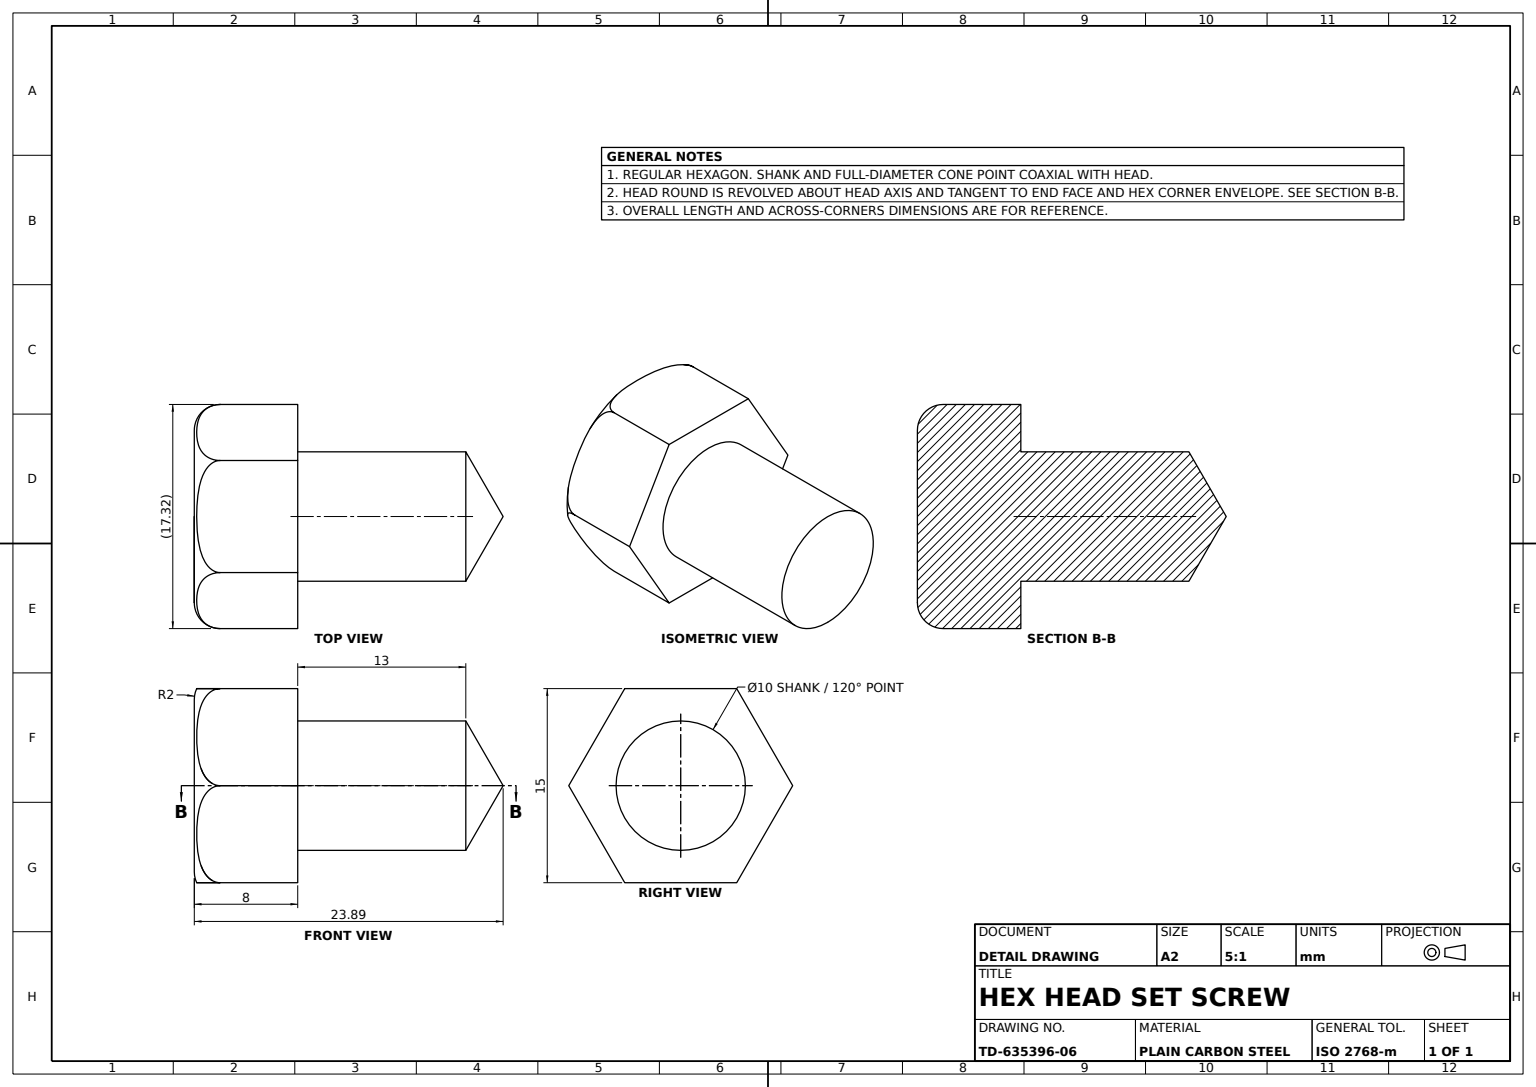
ISO-10303-21;
HEADER;
FILE_DESCRIPTION((''),'2;1');
FILE_NAME('','',(''),(''),'','','');
FILE_SCHEMA(('AUTOMOTIVE_DESIGN'));
ENDSEC;
DATA;
#1=APPLICATION_CONTEXT('');
#2=PRODUCT_CONTEXT('',#1,'mechanical');
#3=PRODUCT('','','',(#2));
#4=PRODUCT_DEFINITION_FORMATION('','',#3);
#5=PRODUCT_DEFINITION_CONTEXT('',#1,'design');
#6=PRODUCT_DEFINITION('','',#4,#5);
#7=PRODUCT_DEFINITION_SHAPE('','',#6);
#8=(LENGTH_UNIT()NAMED_UNIT(*)SI_UNIT(.MILLI.,.METRE.));
#9=(NAMED_UNIT(*)PLANE_ANGLE_UNIT()SI_UNIT($,.RADIAN.));
#10=(NAMED_UNIT(*)SI_UNIT($,.STERADIAN.)SOLID_ANGLE_UNIT());
#11=UNCERTAINTY_MEASURE_WITH_UNIT(LENGTH_MEASURE(1.E-05),#8,'distance_accuracy_value','');
#12=(GEOMETRIC_REPRESENTATION_CONTEXT(3)GLOBAL_UNCERTAINTY_ASSIGNED_CONTEXT((#11))GLOBAL_UNIT_ASSIGNED_CONTEXT((#8,#9,#10))REPRESENTATION_CONTEXT('',''));
#13=CARTESIAN_POINT('',(-8.660254,8.,0.));
#14=VERTEX_POINT('',#13);
#15=CARTESIAN_POINT('',(-8.660254,2.,0.));
#16=VERTEX_POINT('',#15);
#17=DIRECTION('',(0.,-1.,0.));
#18=VECTOR('',#17,1000.);
#19=LINE('',#13,#18);
#20=EDGE_CURVE('',#14,#16,#19,.T.);
#21=ORIENTED_EDGE('',*,*,#20,.T.);
#22=CARTESIAN_POINT('',(-4.330127,2.,7.5));
#23=VERTEX_POINT('',#22);
#24=CARTESIAN_POINT('',(-8.660254,1.782889,0.));
#25=CARTESIAN_POINT('',(-8.623784,1.57369,0.063167));
#26=CARTESIAN_POINT('',(-8.505324,1.213826,0.268346));
#27=CARTESIAN_POINT('',(-8.426378,1.065628,0.405084));
#28=CARTESIAN_POINT('',(-8.25053,0.816976,0.709662));
#29=CARTESIAN_POINT('',(-8.155992,0.719501,0.873407));
#30=CARTESIAN_POINT('',(-7.959026,0.556585,1.214562));
#31=CARTESIAN_POINT('',(-7.856201,0.491675,1.39266));
#32=CARTESIAN_POINT('',(-7.547724,0.334421,1.926959));
#33=CARTESIAN_POINT('',(-7.338836,0.275448,2.288763));
#34=CARTESIAN_POINT('',(-6.918046,0.200226,3.017593));
#35=CARTESIAN_POINT('',(-6.705496,0.184745,3.38574));
#36=CARTESIAN_POINT('',(-6.281467,0.184924,4.120181));
#37=CARTESIAN_POINT('',(-6.070037,0.200451,4.486388));
#38=CARTESIAN_POINT('',(-5.648866,0.276115,5.215877));
#39=CARTESIAN_POINT('',(-5.437857,0.335986,5.581356));
#40=CARTESIAN_POINT('',(-5.128385,0.495087,6.117376));
#41=CARTESIAN_POINT('',(-5.026583,0.559904,6.293703));
#42=CARTESIAN_POINT('',(-4.829796,0.723958,6.634548));
#43=CARTESIAN_POINT('',(-4.735766,0.82189,6.797412));
#44=CARTESIAN_POINT('',(-4.561902,1.06949,7.098554));
#45=CARTESIAN_POINT('',(-4.482703,1.219577,7.23573));
#46=CARTESIAN_POINT('',(-4.39537,1.487005,7.386996));
#47=CARTESIAN_POINT('',(-4.371928,1.581655,7.427598));
#48=CARTESIAN_POINT('',(-4.339075,1.784588,7.484502));
#49=CARTESIAN_POINT('',(-4.330127,1.891998,7.5));
#50=B_SPLINE_CURVE_WITH_KNOTS('',3,(#15,#24,#25,#26,#27,#28,#29,#30,#31,#32,#33,#34,#35,#36,#37,#38,#39,#40,#41,#42,#43,#44,#45,#46,#47,#48,#49,#22),.UNSPECIFIED.,.F.,.F.,(4,2,2,2,2,2,2,2,2,2,2,2,2,4),(0.000000197,0.000641692,0.001283186,0.001924681,0.002566175,0.003849164,0.005132153,0.006415143,0.007698132,0.008339626,0.008981121,0.009622615,0.009943363,0.01026411),.UNSPECIFIED.);
#51=EDGE_CURVE('',#16,#23,#50,.T.);
#52=ORIENTED_EDGE('',*,*,#51,.T.);
#53=CARTESIAN_POINT('',(-4.330127,8.,7.5));
#54=VERTEX_POINT('',#53);
#55=LINE('',#53,#18);
#56=EDGE_CURVE('',#54,#23,#55,.T.);
#57=ORIENTED_EDGE('',*,*,#56,.F.);
#58=DIRECTION('',(0.5,0.,0.866025404));
#59=VECTOR('',#58,1000.);
#60=LINE('',#13,#59);
#61=EDGE_CURVE('',#14,#54,#60,.T.);
#62=ORIENTED_EDGE('',*,*,#61,.F.);
#63=EDGE_LOOP('',(#21,#52,#57,#62));
#64=FACE_OUTER_BOUND('',#63,.T.);
#65=DIRECTION('',(0.866025404,0.,-0.5));
#66=DIRECTION('',(-0.5,0.,-0.866025404));
#67=AXIS2_PLACEMENT_3D('',#13,#65,#66);
#68=PLANE('',#67);
#69=ADVANCED_FACE('',(#64),#68,.F.);
#70=CARTESIAN_POINT('',(8.660254,8.,0.));
#71=VERTEX_POINT('',#70);
#72=CARTESIAN_POINT('',(4.330127,8.,-7.5));
#73=VERTEX_POINT('',#72);
#74=VECTOR('',#66,1000.);
#75=LINE('',#70,#74);
#76=EDGE_CURVE('',#71,#73,#75,.T.);
#77=ORIENTED_EDGE('',*,*,#76,.F.);
#78=CARTESIAN_POINT('',(8.660254,2.,0.));
#79=VERTEX_POINT('',#78);
#80=LINE('',#70,#18);
#81=EDGE_CURVE('',#71,#79,#80,.T.);
#82=ORIENTED_EDGE('',*,*,#81,.T.);
#83=CARTESIAN_POINT('',(4.330127,2.,-7.5));
#84=VERTEX_POINT('',#83);
#85=CARTESIAN_POINT('',(8.660254,1.782889,0.));
#86=CARTESIAN_POINT('',(8.623784,1.57369,-0.063167));
#87=CARTESIAN_POINT('',(8.505324,1.213826,-0.268346));
#88=CARTESIAN_POINT('',(8.426378,1.065628,-0.405084));
#89=CARTESIAN_POINT('',(8.25053,0.816976,-0.709662));
#90=CARTESIAN_POINT('',(8.155992,0.719501,-0.873407));
#91=CARTESIAN_POINT('',(7.959026,0.556585,-1.214562));
#92=CARTESIAN_POINT('',(7.856201,0.491675,-1.39266));
#93=CARTESIAN_POINT('',(7.547724,0.334421,-1.926959));
#94=CARTESIAN_POINT('',(7.338836,0.275448,-2.288763));
#95=CARTESIAN_POINT('',(6.918046,0.200226,-3.017593));
#96=CARTESIAN_POINT('',(6.705496,0.184745,-3.38574));
#97=CARTESIAN_POINT('',(6.281467,0.184924,-4.120181));
#98=CARTESIAN_POINT('',(6.070037,0.200451,-4.486388));
#99=CARTESIAN_POINT('',(5.648866,0.276115,-5.215877));
#100=CARTESIAN_POINT('',(5.437857,0.335986,-5.581356));
#101=CARTESIAN_POINT('',(5.128385,0.495087,-6.117376));
#102=CARTESIAN_POINT('',(5.026583,0.559904,-6.293703));
#103=CARTESIAN_POINT('',(4.829796,0.723958,-6.634548));
#104=CARTESIAN_POINT('',(4.735766,0.82189,-6.797412));
#105=CARTESIAN_POINT('',(4.561902,1.06949,-7.098554));
#106=CARTESIAN_POINT('',(4.482703,1.219577,-7.23573));
#107=CARTESIAN_POINT('',(4.39537,1.487005,-7.386996));
#108=CARTESIAN_POINT('',(4.371928,1.581655,-7.427598));
#109=CARTESIAN_POINT('',(4.339075,1.784588,-7.484502));
#110=CARTESIAN_POINT('',(4.330127,1.891998,-7.5));
#111=B_SPLINE_CURVE_WITH_KNOTS('',3,(#78,#85,#86,#87,#88,#89,#90,#91,#92,#93,#94,#95,#96,#97,#98,#99,#100,#101,#102,#103,#104,#105,#106,#107,#108,#109,#110,#83),.UNSPECIFIED.,.F.,.F.,(4,2,2,2,2,2,2,2,2,2,2,2,2,4),(0.000000197,0.000641692,0.001283186,0.001924681,0.002566175,0.003849164,0.005132153,0.006415143,0.007698132,0.008339626,0.008981121,0.009622615,0.009943363,0.01026411),.UNSPECIFIED.);
#112=EDGE_CURVE('',#79,#84,#111,.T.);
#113=ORIENTED_EDGE('',*,*,#112,.T.);
#114=LINE('',#72,#18);
#115=EDGE_CURVE('',#73,#84,#114,.T.);
#116=ORIENTED_EDGE('',*,*,#115,.F.);
#117=EDGE_LOOP('',(#77,#82,#113,#116));
#118=FACE_OUTER_BOUND('',#117,.T.);
#119=DIRECTION('',(-0.866025404,0.,0.5));
#120=AXIS2_PLACEMENT_3D('',#70,#119,#58);
#121=PLANE('',#120);
#122=ADVANCED_FACE('',(#118),#121,.F.);
#123=CARTESIAN_POINT('',(0.,21.,-5.));
#124=VERTEX_POINT('',#123);
#125=CARTESIAN_POINT('',(0.,21.,5.));
#126=VERTEX_POINT('',#125);
#127=CARTESIAN_POINT('',(0.,21.,0.));
#128=DIRECTION('',(0.,0.,-1.));
#129=AXIS2_PLACEMENT_3D('',#127,#17,#128);
#130=CIRCLE('',#129,5.);
#131=EDGE_CURVE('',#124,#126,#130,.T.);
#132=ORIENTED_EDGE('',*,*,#131,.F.);
#133=CARTESIAN_POINT('',(0.,23.886751,0.));
#134=VERTEX_POINT('',#133);
#135=DIRECTION('',(0.,-0.5,-0.866025404));
#136=VECTOR('',#135,1000.);
#137=LINE('',#123,#136);
#138=EDGE_CURVE('',#134,#124,#137,.T.);
#139=ORIENTED_EDGE('',*,*,#138,.F.);
#140=DIRECTION('',(0.,-0.5,0.866025404));
#141=VECTOR('',#140,1000.);
#142=LINE('',#125,#141);
#143=EDGE_CURVE('',#134,#126,#142,.T.);
#144=ORIENTED_EDGE('',*,*,#143,.T.);
#145=EDGE_LOOP('',(#132,#139,#144));
#146=FACE_OUTER_BOUND('',#145,.T.);
#147=CONICAL_SURFACE('',#129,5.,1.047197551);
#148=ADVANCED_FACE('',(#146),#147,.T.);
#149=ORIENTED_EDGE('',*,*,#143,.F.);
#150=ORIENTED_EDGE('',*,*,#138,.T.);
#151=EDGE_CURVE('',#126,#124,#130,.T.);
#152=ORIENTED_EDGE('',*,*,#151,.F.);
#153=EDGE_LOOP('',(#149,#150,#152));
#154=FACE_OUTER_BOUND('',#153,.T.);
#155=ADVANCED_FACE('',(#154),#147,.T.);
#156=CARTESIAN_POINT('',(0.,8.,-5.));
#157=VERTEX_POINT('',#156);
#158=CARTESIAN_POINT('',(0.,23.886751,-5.));
#159=LINE('',#158,#18);
#160=EDGE_CURVE('',#124,#157,#159,.T.);
#161=ORIENTED_EDGE('',*,*,#160,.F.);
#162=ORIENTED_EDGE('',*,*,#131,.T.);
#163=CARTESIAN_POINT('',(0.,8.,5.));
#164=VERTEX_POINT('',#163);
#165=CARTESIAN_POINT('',(0.,23.886751,5.));
#166=LINE('',#165,#18);
#167=EDGE_CURVE('',#126,#164,#166,.T.);
#168=ORIENTED_EDGE('',*,*,#167,.T.);
#169=CARTESIAN_POINT('',(0.,8.,0.));
#170=AXIS2_PLACEMENT_3D('',#169,#17,#128);
#171=CIRCLE('',#170,5.);
#172=EDGE_CURVE('',#157,#164,#171,.T.);
#173=ORIENTED_EDGE('',*,*,#172,.F.);
#174=EDGE_LOOP('',(#161,#162,#168,#173));
#175=FACE_OUTER_BOUND('',#174,.T.);
#176=AXIS2_PLACEMENT_3D('',#133,#17,#128);
#177=CYLINDRICAL_SURFACE('',#176,5.);
#178=ADVANCED_FACE('',(#175),#177,.T.);
#179=CARTESIAN_POINT('',(-4.330127,8.,-7.5));
#180=VERTEX_POINT('',#179);
#181=CARTESIAN_POINT('',(-4.330127,2.,-7.5));
#182=VERTEX_POINT('',#181);
#183=LINE('',#179,#18);
#184=EDGE_CURVE('',#180,#182,#183,.T.);
#185=ORIENTED_EDGE('',*,*,#184,.T.);
#186=CARTESIAN_POINT('',(-4.330127,1.782889,-7.5));
#187=CARTESIAN_POINT('',(-4.366597,1.57369,-7.436833));
#188=CARTESIAN_POINT('',(-4.485057,1.213826,-7.231654));
#189=CARTESIAN_POINT('',(-4.564003,1.065628,-7.094916));
#190=CARTESIAN_POINT('',(-4.739851,0.816976,-6.790338));
#191=CARTESIAN_POINT('',(-4.834389,0.719501,-6.626593));
#192=CARTESIAN_POINT('',(-5.031355,0.556585,-6.285438));
#193=CARTESIAN_POINT('',(-5.13418,0.491675,-6.10734));
#194=CARTESIAN_POINT('',(-5.442657,0.334421,-5.573041));
#195=CARTESIAN_POINT('',(-5.651545,0.275448,-5.211237));
#196=CARTESIAN_POINT('',(-6.072335,0.200226,-4.482407));
#197=CARTESIAN_POINT('',(-6.284885,0.184745,-4.11426));
#198=CARTESIAN_POINT('',(-6.708914,0.184924,-3.379819));
#199=CARTESIAN_POINT('',(-6.920344,0.200451,-3.013612));
#200=CARTESIAN_POINT('',(-7.341515,0.276115,-2.284123));
#201=CARTESIAN_POINT('',(-7.552524,0.335986,-1.918644));
#202=CARTESIAN_POINT('',(-7.861996,0.495087,-1.382624));
#203=CARTESIAN_POINT('',(-7.963798,0.559904,-1.206297));
#204=CARTESIAN_POINT('',(-8.160585,0.723958,-0.865452));
#205=CARTESIAN_POINT('',(-8.254615,0.82189,-0.702588));
#206=CARTESIAN_POINT('',(-8.428479,1.06949,-0.401446));
#207=CARTESIAN_POINT('',(-8.507678,1.219577,-0.26427));
#208=CARTESIAN_POINT('',(-8.595011,1.487005,-0.113004));
#209=CARTESIAN_POINT('',(-8.618453,1.581655,-0.072402));
#210=CARTESIAN_POINT('',(-8.651307,1.784588,-0.015498));
#211=CARTESIAN_POINT('',(-8.660254,1.891998,0.));
#212=B_SPLINE_CURVE_WITH_KNOTS('',3,(#181,#186,#187,#188,#189,#190,#191,#192,#193,#194,#195,#196,#197,#198,#199,#200,#201,#202,#203,#204,#205,#206,#207,#208,#209,#210,#211,#15),.UNSPECIFIED.,.F.,.F.,(4,2,2,2,2,2,2,2,2,2,2,2,2,4),(0.000000197,0.000641692,0.001283186,0.001924681,0.002566175,0.003849164,0.005132153,0.006415143,0.007698132,0.008339626,0.008981121,0.009622615,0.009943363,0.01026411),.UNSPECIFIED.);
#213=EDGE_CURVE('',#182,#16,#212,.T.);
#214=ORIENTED_EDGE('',*,*,#213,.T.);
#215=ORIENTED_EDGE('',*,*,#20,.F.);
#216=DIRECTION('',(-0.5,0.,0.866025404));
#217=VECTOR('',#216,1000.);
#218=LINE('',#179,#217);
#219=EDGE_CURVE('',#180,#14,#218,.T.);
#220=ORIENTED_EDGE('',*,*,#219,.F.);
#221=EDGE_LOOP('',(#185,#214,#215,#220));
#222=FACE_OUTER_BOUND('',#221,.T.);
#223=DIRECTION('',(0.866025404,0.,0.5));
#224=DIRECTION('',(0.5,0.,-0.866025404));
#225=AXIS2_PLACEMENT_3D('',#179,#223,#224);
#226=PLANE('',#225);
#227=ADVANCED_FACE('',(#222),#226,.F.);
#228=CARTESIAN_POINT('',(4.330127,8.,7.5));
#229=VERTEX_POINT('',#228);
#230=VECTOR('',#224,1000.);
#231=LINE('',#228,#230);
#232=EDGE_CURVE('',#229,#71,#231,.T.);
#233=ORIENTED_EDGE('',*,*,#232,.T.);
#234=ORIENTED_EDGE('',*,*,#76,.T.);
#235=DIRECTION('',(-1.,0.,0.));
#236=VECTOR('',#235,1000.);
#237=LINE('',#72,#236);
#238=EDGE_CURVE('',#73,#180,#237,.T.);
#239=ORIENTED_EDGE('',*,*,#238,.T.);
#240=ORIENTED_EDGE('',*,*,#219,.T.);
#241=ORIENTED_EDGE('',*,*,#61,.T.);
#242=DIRECTION('',(1.,0.,0.));
#243=VECTOR('',#242,1000.);
#244=LINE('',#53,#243);
#245=EDGE_CURVE('',#54,#229,#244,.T.);
#246=ORIENTED_EDGE('',*,*,#245,.T.);
#247=EDGE_LOOP('',(#233,#234,#239,#240,#241,#246));
#248=FACE_OUTER_BOUND('',#247,.T.);
#249=EDGE_CURVE('',#164,#157,#171,.T.);
#250=ORIENTED_EDGE('',*,*,#249,.T.);
#251=ORIENTED_EDGE('',*,*,#172,.T.);
#252=EDGE_LOOP('',(#250,#251));
#253=FACE_BOUND('',#252,.T.);
#254=DIRECTION('',(0.,1.,0.));
#255=DIRECTION('',(0.,0.,1.));
#256=AXIS2_PLACEMENT_3D('',#169,#254,#255);
#257=PLANE('',#256);
#258=ADVANCED_FACE('',(#248,#253),#257,.T.);
#259=CARTESIAN_POINT('',(0.,0.184834,7.5));
#260=VERTEX_POINT('',#259);
#261=CARTESIAN_POINT('',(0.,0.,6.660254));
#262=VERTEX_POINT('',#261);
#263=CARTESIAN_POINT('',(0.,2.,6.660254));
#264=AXIS2_PLACEMENT_3D('',#263,#242,#128);
#265=CIRCLE('',#264,2.);
#266=EDGE_CURVE('',#260,#262,#265,.T.);
#267=ORIENTED_EDGE('',*,*,#266,.F.);
#268=CARTESIAN_POINT('',(-4.330127,1.893334,7.5));
#269=CARTESIAN_POINT('',(-4.312428,1.785382,7.5));
#270=CARTESIAN_POINT('',(-4.24669,1.581979,7.5));
#271=CARTESIAN_POINT('',(-4.198141,1.484258,7.5));
#272=CARTESIAN_POINT('',(-4.081248,1.3062,7.5));
#273=CARTESIAN_POINT('',(-4.01173,1.223551,7.5));
#274=CARTESIAN_POINT('',(-3.8593,1.073065,7.5));
#275=CARTESIAN_POINT('',(-3.777137,1.00565,7.5));
#276=CARTESIAN_POINT('',(-3.517234,0.821056,7.5));
#277=CARTESIAN_POINT('',(-3.325251,0.721345,7.5));
#278=CARTESIAN_POINT('',(-2.933762,0.558776,7.5));
#279=CARTESIAN_POINT('',(-2.731909,0.494598,7.5));
#280=CARTESIAN_POINT('',(-2.320129,0.388853,7.5));
#281=CARTESIAN_POINT('',(-2.110361,0.347561,7.5));
#282=CARTESIAN_POINT('',(-1.691288,0.281775,7.5));
#283=CARTESIAN_POINT('',(-1.481011,0.257081,7.5));
#284=CARTESIAN_POINT('',(-0.848617,0.200347,7.5));
#285=CARTESIAN_POINT('',(-0.427033,0.184834,7.5));
#286=B_SPLINE_CURVE_WITH_KNOTS('',3,(#22,#268,#269,#270,#271,#272,#273,#274,#275,#276,#277,#278,#279,#280,#281,#282,#283,#284,#285,#259),.UNSPECIFIED.,.F.,.F.,(4,2,2,2,2,2,2,2,2,4),(0.015324776,0.015644365,0.015963954,0.016283543,0.016603132,0.01724231,0.017881488,0.018520667,0.019159845,0.020438201),.UNSPECIFIED.);
#287=EDGE_CURVE('',#23,#260,#286,.T.);
#288=ORIENTED_EDGE('',*,*,#287,.F.);
#289=ORIENTED_EDGE('',*,*,#51,.F.);
#290=ORIENTED_EDGE('',*,*,#213,.F.);
#291=CARTESIAN_POINT('',(0.,0.184834,-7.5));
#292=VERTEX_POINT('',#291);
#293=CARTESIAN_POINT('',(-0.425292,0.184834,-7.5));
#294=CARTESIAN_POINT('',(-0.849566,0.200351,-7.5));
#295=CARTESIAN_POINT('',(-1.695166,0.276374,-7.5));
#296=CARTESIAN_POINT('',(-2.118525,0.336921,-7.5));
#297=CARTESIAN_POINT('',(-2.732724,0.494888,-7.5));
#298=CARTESIAN_POINT('',(-2.934319,0.558905,-7.5));
#299=CARTESIAN_POINT('',(-3.327696,0.722463,-7.5));
#300=CARTESIAN_POINT('',(-3.518535,0.821654,-7.5));
#301=CARTESIAN_POINT('',(-3.867059,1.069846,-7.5));
#302=CARTESIAN_POINT('',(-4.022715,1.216544,-7.5));
#303=CARTESIAN_POINT('',(-4.19958,1.4867,-7.5));
#304=CARTESIAN_POINT('',(-4.247014,1.582666,-7.5));
#305=CARTESIAN_POINT('',(-4.312716,1.786593,-7.5));
#306=CARTESIAN_POINT('',(-4.330127,1.893579,-7.5));
#307=B_SPLINE_CURVE_WITH_KNOTS('',3,(#291,#293,#294,#295,#296,#297,#298,#299,#300,#301,#302,#303,#304,#305,#306,#181),.UNSPECIFIED.,.F.,.F.,(4,2,2,2,2,2,2,4),(0.,0.001273142,0.002546285,0.003182856,0.003819427,0.004455999,0.004774284,0.00509257),.UNSPECIFIED.);
#308=EDGE_CURVE('',#292,#182,#307,.T.);
#309=ORIENTED_EDGE('',*,*,#308,.F.);
#310=CARTESIAN_POINT('',(0.,0.,-6.660254));
#311=VERTEX_POINT('',#310);
#312=CARTESIAN_POINT('',(0.,2.,-6.660254));
#313=AXIS2_PLACEMENT_3D('',#312,#235,#255);
#314=CIRCLE('',#313,2.);
#315=EDGE_CURVE('',#292,#311,#314,.T.);
#316=ORIENTED_EDGE('',*,*,#315,.T.);
#317=CARTESIAN_POINT('',(0.,0.,0.));
#318=AXIS2_PLACEMENT_3D('',#317,#17,#128);
#319=CIRCLE('',#318,6.660254);
#320=EDGE_CURVE('',#262,#311,#319,.T.);
#321=ORIENTED_EDGE('',*,*,#320,.F.);
#322=EDGE_LOOP('',(#267,#288,#289,#290,#309,#316,#321));
#323=FACE_OUTER_BOUND('',#322,.T.);
#324=CARTESIAN_POINT('',(0.,2.,0.));
#325=AXIS2_PLACEMENT_3D('',#324,#17,#128);
#326=TOROIDAL_SURFACE('',#325,6.660254,2.);
#327=ADVANCED_FACE('',(#323),#326,.T.);
#328=ORIENTED_EDGE('',*,*,#56,.T.);
#329=ORIENTED_EDGE('',*,*,#287,.T.);
#330=CARTESIAN_POINT('',(4.330127,2.,7.5));
#331=VERTEX_POINT('',#330);
#332=CARTESIAN_POINT('',(0.425292,0.184834,7.5));
#333=CARTESIAN_POINT('',(0.849566,0.200351,7.5));
#334=CARTESIAN_POINT('',(1.695166,0.276374,7.5));
#335=CARTESIAN_POINT('',(2.118525,0.336921,7.5));
#336=CARTESIAN_POINT('',(2.732724,0.494888,7.5));
#337=CARTESIAN_POINT('',(2.934319,0.558905,7.5));
#338=CARTESIAN_POINT('',(3.327696,0.722463,7.5));
#339=CARTESIAN_POINT('',(3.518535,0.821654,7.5));
#340=CARTESIAN_POINT('',(3.867059,1.069846,7.5));
#341=CARTESIAN_POINT('',(4.022715,1.216544,7.5));
#342=CARTESIAN_POINT('',(4.19958,1.4867,7.5));
#343=CARTESIAN_POINT('',(4.247014,1.582666,7.5));
#344=CARTESIAN_POINT('',(4.312716,1.786593,7.5));
#345=CARTESIAN_POINT('',(4.330127,1.893579,7.5));
#346=B_SPLINE_CURVE_WITH_KNOTS('',3,(#259,#332,#333,#334,#335,#336,#337,#338,#339,#340,#341,#342,#343,#344,#345,#330),.UNSPECIFIED.,.F.,.F.,(4,2,2,2,2,2,2,4),(0.,0.001273142,0.002546285,0.003182856,0.003819427,0.004455999,0.004774284,0.00509257),.UNSPECIFIED.);
#347=EDGE_CURVE('',#260,#331,#346,.T.);
#348=ORIENTED_EDGE('',*,*,#347,.T.);
#349=LINE('',#228,#18);
#350=EDGE_CURVE('',#229,#331,#349,.T.);
#351=ORIENTED_EDGE('',*,*,#350,.F.);
#352=ORIENTED_EDGE('',*,*,#245,.F.);
#353=EDGE_LOOP('',(#328,#329,#348,#351,#352));
#354=FACE_OUTER_BOUND('',#353,.T.);
#355=AXIS2_PLACEMENT_3D('',#53,#128,#235);
#356=PLANE('',#355);
#357=ADVANCED_FACE('',(#354),#356,.F.);
#358=ORIENTED_EDGE('',*,*,#266,.T.);
#359=EDGE_CURVE('',#311,#262,#319,.T.);
#360=ORIENTED_EDGE('',*,*,#359,.F.);
#361=ORIENTED_EDGE('',*,*,#315,.F.);
#362=CARTESIAN_POINT('',(4.330127,1.893334,-7.5));
#363=CARTESIAN_POINT('',(4.312428,1.785382,-7.5));
#364=CARTESIAN_POINT('',(4.24669,1.581979,-7.5));
#365=CARTESIAN_POINT('',(4.198141,1.484258,-7.5));
#366=CARTESIAN_POINT('',(4.081248,1.3062,-7.5));
#367=CARTESIAN_POINT('',(4.01173,1.223551,-7.5));
#368=CARTESIAN_POINT('',(3.8593,1.073065,-7.5));
#369=CARTESIAN_POINT('',(3.777137,1.00565,-7.5));
#370=CARTESIAN_POINT('',(3.517234,0.821056,-7.5));
#371=CARTESIAN_POINT('',(3.325251,0.721345,-7.5));
#372=CARTESIAN_POINT('',(2.933762,0.558776,-7.5));
#373=CARTESIAN_POINT('',(2.731909,0.494598,-7.5));
#374=CARTESIAN_POINT('',(2.320129,0.388853,-7.5));
#375=CARTESIAN_POINT('',(2.110361,0.347561,-7.5));
#376=CARTESIAN_POINT('',(1.691288,0.281775,-7.5));
#377=CARTESIAN_POINT('',(1.481011,0.257081,-7.5));
#378=CARTESIAN_POINT('',(0.848617,0.200347,-7.5));
#379=CARTESIAN_POINT('',(0.427033,0.184834,-7.5));
#380=B_SPLINE_CURVE_WITH_KNOTS('',3,(#83,#362,#363,#364,#365,#366,#367,#368,#369,#370,#371,#372,#373,#374,#375,#376,#377,#378,#379,#291),.UNSPECIFIED.,.F.,.F.,(4,2,2,2,2,2,2,2,2,4),(0.015324776,0.015644365,0.015963954,0.016283543,0.016603132,0.01724231,0.017881488,0.018520667,0.019159845,0.020438201),.UNSPECIFIED.);
#381=EDGE_CURVE('',#84,#292,#380,.T.);
#382=ORIENTED_EDGE('',*,*,#381,.F.);
#383=ORIENTED_EDGE('',*,*,#112,.F.);
#384=CARTESIAN_POINT('',(4.330127,1.782889,7.5));
#385=CARTESIAN_POINT('',(4.366597,1.57369,7.436833));
#386=CARTESIAN_POINT('',(4.485057,1.213826,7.231654));
#387=CARTESIAN_POINT('',(4.564003,1.065628,7.094916));
#388=CARTESIAN_POINT('',(4.739851,0.816976,6.790338));
#389=CARTESIAN_POINT('',(4.834389,0.719501,6.626593));
#390=CARTESIAN_POINT('',(5.031355,0.556585,6.285438));
#391=CARTESIAN_POINT('',(5.13418,0.491675,6.10734));
#392=CARTESIAN_POINT('',(5.442657,0.334421,5.573041));
#393=CARTESIAN_POINT('',(5.651545,0.275448,5.211237));
#394=CARTESIAN_POINT('',(6.072335,0.200226,4.482407));
#395=CARTESIAN_POINT('',(6.284885,0.184745,4.11426));
#396=CARTESIAN_POINT('',(6.708914,0.184924,3.379819));
#397=CARTESIAN_POINT('',(6.920344,0.200451,3.013612));
#398=CARTESIAN_POINT('',(7.341515,0.276115,2.284123));
#399=CARTESIAN_POINT('',(7.552524,0.335986,1.918644));
#400=CARTESIAN_POINT('',(7.861996,0.495087,1.382624));
#401=CARTESIAN_POINT('',(7.963798,0.559904,1.206297));
#402=CARTESIAN_POINT('',(8.160585,0.723958,0.865452));
#403=CARTESIAN_POINT('',(8.254615,0.82189,0.702588));
#404=CARTESIAN_POINT('',(8.428479,1.06949,0.401446));
#405=CARTESIAN_POINT('',(8.507678,1.219577,0.26427));
#406=CARTESIAN_POINT('',(8.595011,1.487005,0.113004));
#407=CARTESIAN_POINT('',(8.618453,1.581655,0.072402));
#408=CARTESIAN_POINT('',(8.651307,1.784588,0.015498));
#409=CARTESIAN_POINT('',(8.660254,1.891998,0.));
#410=B_SPLINE_CURVE_WITH_KNOTS('',3,(#330,#384,#385,#386,#387,#388,#389,#390,#391,#392,#393,#394,#395,#396,#397,#398,#399,#400,#401,#402,#403,#404,#405,#406,#407,#408,#409,#78),.UNSPECIFIED.,.F.,.F.,(4,2,2,2,2,2,2,2,2,2,2,2,2,4),(0.000000197,0.000641692,0.001283186,0.001924681,0.002566175,0.003849164,0.005132153,0.006415143,0.007698132,0.008339626,0.008981121,0.009622615,0.009943363,0.01026411),.UNSPECIFIED.);
#411=EDGE_CURVE('',#331,#79,#410,.T.);
#412=ORIENTED_EDGE('',*,*,#411,.F.);
#413=ORIENTED_EDGE('',*,*,#347,.F.);
#414=EDGE_LOOP('',(#358,#360,#361,#382,#383,#412,#413));
#415=FACE_OUTER_BOUND('',#414,.T.);
#416=ADVANCED_FACE('',(#415),#326,.T.);
#417=ORIENTED_EDGE('',*,*,#151,.T.);
#418=ORIENTED_EDGE('',*,*,#160,.T.);
#419=ORIENTED_EDGE('',*,*,#249,.F.);
#420=ORIENTED_EDGE('',*,*,#167,.F.);
#421=EDGE_LOOP('',(#417,#418,#419,#420));
#422=FACE_OUTER_BOUND('',#421,.T.);
#423=ADVANCED_FACE('',(#422),#177,.T.);
#424=ORIENTED_EDGE('',*,*,#232,.F.);
#425=ORIENTED_EDGE('',*,*,#350,.T.);
#426=ORIENTED_EDGE('',*,*,#411,.T.);
#427=ORIENTED_EDGE('',*,*,#81,.F.);
#428=EDGE_LOOP('',(#424,#425,#426,#427));
#429=FACE_OUTER_BOUND('',#428,.T.);
#430=DIRECTION('',(-0.866025404,0.,-0.5));
#431=AXIS2_PLACEMENT_3D('',#228,#430,#216);
#432=PLANE('',#431);
#433=ADVANCED_FACE('',(#429),#432,.F.);
#434=ORIENTED_EDGE('',*,*,#381,.T.);
#435=ORIENTED_EDGE('',*,*,#308,.T.);
#436=ORIENTED_EDGE('',*,*,#184,.F.);
#437=ORIENTED_EDGE('',*,*,#238,.F.);
#438=ORIENTED_EDGE('',*,*,#115,.T.);
#439=EDGE_LOOP('',(#434,#435,#436,#437,#438));
#440=FACE_OUTER_BOUND('',#439,.T.);
#441=AXIS2_PLACEMENT_3D('',#72,#255,#242);
#442=PLANE('',#441);
#443=ADVANCED_FACE('',(#440),#442,.F.);
#444=ORIENTED_EDGE('',*,*,#359,.T.);
#445=ORIENTED_EDGE('',*,*,#320,.T.);
#446=EDGE_LOOP('',(#444,#445));
#447=FACE_OUTER_BOUND('',#446,.T.);
#448=AXIS2_PLACEMENT_3D('',#317,#254,#255);
#449=PLANE('',#448);
#450=ADVANCED_FACE('',(#447),#449,.F.);
#451=CLOSED_SHELL('',(#69,#122,#148,#155,#178,#227,#258,#327,#357,#416,#423,#433,#443,#450));
#452=MANIFOLD_SOLID_BREP('',#451);
#453=ADVANCED_BREP_SHAPE_REPRESENTATION('',(#452),#12);
#454=SHAPE_DEFINITION_REPRESENTATION(#7,#453);
ENDSEC;
END-ISO-10303-21;
